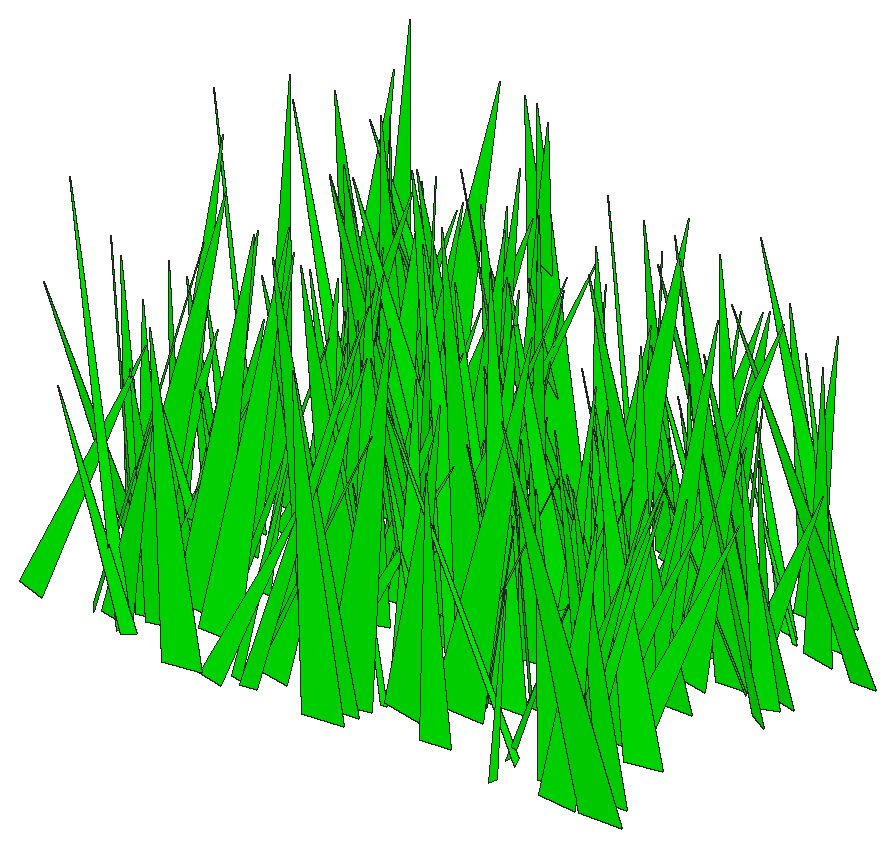
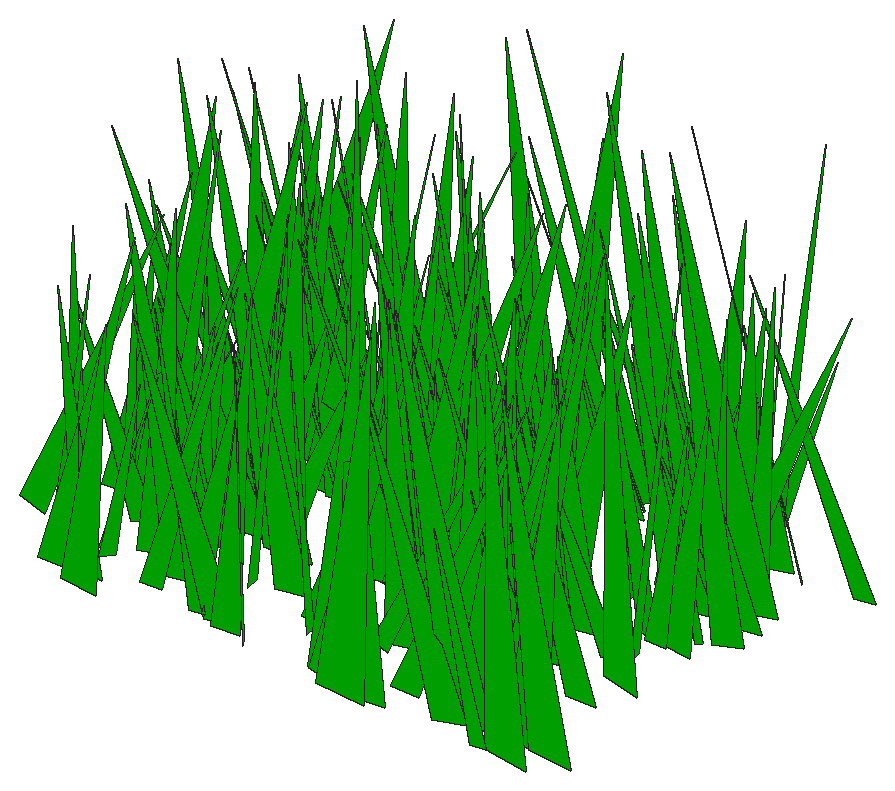
# SketchUp Ruby script. Lengths in inches.
U = 1.inch
M = Sketchup.active_model
def pt(a) = Geom::Point3d.new(a.map { |v| v * U })
def face(e, loops, mat)
  f = e.add_face(loops[0].map { |a| pt(a) })
  loops[1..].each { |l| e.add_face(l.map { |a| pt(a) }).erase! }
  f.material = f.back_material = mat if mat
  f
end
# faces: each face lists its corners as indices into pts; further lists are holes
def faces(e, pts, list, mat = nil) = list.each { |f| face(e, (f[0].is_a?(Array) ? f : [f]).map { |l| l.map { |i| pts[i] } }, mat) }
# xy, xz, yz: faces in a plane at the given z, y or x. An outline is a flat list of corners, or four numbers for a rectangle; further outlines are holes
def ring(l) = l.size == 4 ? [[l[0], l[1]], [l[2], l[1]], [l[2], l[3]], [l[0], l[3]]] : l.each_slice(2).to_a
def flat(e, list, mat, &to3) = list.each { |f| face(e, (f[0].is_a?(Array) ? f : [f]).map { |l| ring(l).map { |u, v| to3.(u, v) } }, mat) }
def xy(e, z, list, mat = nil) = flat(e, list, mat) { |x, y| [x, y, z] }
def xz(e, y, list, mat = nil) = flat(e, list, mat) { |x, z| [x, y, z] }
def yz(e, x, list, mat = nil) = flat(e, list, mat) { |y, z| [x, y, z] }
def lines(e, pts, list) = list.each { |a, b| e.add_line(pt(pts[a]), pt(pts[b])) }
# prism: a flat outline (further loops are holes) pulled along v
def prism(e, loops, v, mat = nil)
  f = face(e, loops, mat); d = Geom::Vector3d.new(v.map { |x| x * U })
  f.pushpull(f.normal.samedirection?(d) ? d.length : -d.length)
end
def box(e, o, s, mat = nil) = prism(e, [[o, [o[0] + s[0], o[1], o[2]], [o[0] + s[0], o[1] + s[1], o[2]], [o[0], o[1] + s[1], o[2]]]], [0, 0, s[2]], mat)
def at(x, y, z, deg = 0) = Geom::Transformation.translation(pt([x, y, z])) * Geom::Transformation.rotation(ORIGIN, Z_AXIS, deg.degrees)
def axes(o, x, y, z) = Geom::Transformation.new([*x, 0, *y, 0, *z, 0, *pt(o).to_a, 1])
def part(name) = M.definitions.add(name)
# library, detail: a bought-in or finely detailed component or shape, given as its bounding box
def library(name, o, s) = part(name).tap { |d| box(d.entities, o, s) }
def detail(e, o, s) = box(e.add_group.entities, o, s)
def put(e, d, t, mat = nil) = e.add_instance(d, t).tap { |i| i.material = mat if mat }
def group(e, t, mat = nil) = e.add_group.tap { |g| g.transformation = t; g.material = mat if mat }.entities
root = M.entities
M.materials.add("[0065_Lime]").color = [0, 255, 0]
c1 = part("fur_instance\#9")
p = [[0.8125,0,1.79],[0.67,-0.02,1.48],[0,-0.11,0],[0,0.11,0]]
faces(c1.entities,p,[[0,1,2,3]])
put(root,c1,axes([71.11,32.47,1.48],[1.31504,-1.01474,1.32526],[7.31505,0.21385,0.68416],[-1.1376,0.20206,5.93131]),"[0065_Lime]")
put(root,c1,axes([70.0625,32.63,1.48],[3.16788,1.04057,0.61952],[-7.4056,0.45235,-0.40482],[-0.75859,-0.07058,6.53906]),"[0065_Lime]")
put(root,c1,axes([71.28,25.28,1.48],[-0.49526,-0.70471,1.4178],[5.29109,-0.04513,0.47119],[-0.43981,0.25059,4.072]),"[0065_Lime]")
put(root,c1,axes([71.29,21.32,1.48],[6.28785,0.11215,2.7973],[-0.35978,1.00228,-0.81143],[-3.51199,0.09812,5.0914]),"[0065_Lime]")
put(root,c1,axes([72.81,20.59,1.48],[-4.84312,-0.62522,0.45458],[4.4821,-0.6712,0.6608],[-0.1432,0.13709,5.30862]),"[0065_Lime]")
put(root,c1,axes([71.03,21.84,1.48],[5.05659,-0.53702,2.1019],[3.79865,0.79038,0.72027],[-2.61785,0.10959,5.10514]),"[0065_Lime]")
put(root,c1,axes([68.77,19.51,1.48],[4.73607,0.58974,0.54638],[-4.24651,0.65059,0.82395],[0.17935,-0.16892,5.08094]),"[0065_Lime]")
put(root,c1,axes([71.95,26.32,1.48],[-8.48103,0.12944,2.12396],[-0.61842,-1.24092,0.90029],[2.69894,0.12241,6.8805]),"[0065_Lime]")
put(root,c1,axes([71.07,33.45,1.48],[4.07033,1.04268,1.70118],[-7.52786,0.60923,-0.5954],[-1.66314,-0.20574,6.8584]),"[0065_Lime]")
put(root,c1,axes([70.23,24.1,1.48],[7.45772,-0.59253,2.41896],[4.64223,1.0911,-0.5137],[-2.25262,0.28689,6.94979]),"[0065_Lime]")
put(root,c1,axes([71.17,27.95,1.48],[5.96669,0.87695,2.17628],[-6.27778,0.90317,-0.80728],[-2.58765,-0.16905,6.97663]),"[0065_Lime]")
put(root,c1,axes([72.04,32.25,1.48],[0.25386,-0.75206,1.27851],[5.50134,0.0703,0.66302],[-0.9221,0.21239,4.3076]),"[0065_Lime]")
put(root,c1,axes([72.67,19.22,1.48],[-4.15449,0.31536,0.77462],[-2.40098,-0.57513,-0.67404],[0.42308,-0.16713,3.78127]),"[0065_Lime]")
put(root,c1,axes([71.95,25.34,1.48],[3.10497,-0.43272,1.84859],[3.21889,0.51771,0.48359],[-2.07044,0.15594,3.52411]),"[0065_Lime]")
put(root,c1,axes([71.68,22.82,1.48],[4.8907,0.49632,1.94087],[-3.40285,0.76194,-0.85566],[-2.56705,-0.06443,4.83198]),"[0065_Lime]")
put(root,c1,axes([72.34,19.4,1.48],[-8.64109,0.1221,2.44965],[-1.21349,-1.27456,-0.70341],[2.88998,-0.1701,7.02912]),"[0065_Lime]")
put(root,c1,axes([70.38,23.06,1.48],[0.93197,0.76973,0.26058],[-5.4343,0.12315,0.66989],[0.76009,-0.06333,4.46986]),"[0065_Lime]")
put(root,c1,axes([70.94,31.95,1.48],[0.54433,0.53862,1.59453],[-4.28288,0.03946,0.52074],[0.43863,-0.28314,3.10583]),"[0065_Lime]")
put(root,c1,axes([70.98,24.51,1.48],[3.81899,0.20071,1.17784],[-1.81606,0.5314,0.86171],[-0.91588,-0.21679,3.20267]),"[0065_Lime]")
put(root,c1,axes([70.98,31.86,1.48],[-0.66186,-0.82891,0.88827],[5.88182,-0.12005,-0.85414],[1.18088,0.13336,4.75225]),"[0065_Lime]")
put(root,c1,axes([72.12,32.28,1.48],[-2.30581,0.56203,0.7001],[-3.98197,-0.34017,0.47345],[0.93939,-0.06239,3.72537]),"[0065_Lime]")
put(root,c1,axes([72.6875,20.4,1.48],[1.18339,0.93993,0.30109],[-6.60693,0.17248,-0.8617],[-1.1084,-0.02462,5.45783]),"[0065_Lime]")
put(root,c1,axes([70.65,23.57,1.48],[3.30012,0.38045,0.41179],[-2.74444,0.44474,0.78362],[0.23403,-0.14935,3.38258]),"[0065_Lime]")
put(root,c1,axes([72.34,32.04,1.48],[6.11772,0.32407,2.61673],[-2.78615,0.94364,0.39383],[-2.81158,-0.22997,5.30348]),"[0065_Lime]")
put(root,c1,axes([70.75,22.13,1.48],[5.9783,-0.91796,1.63314],[6.78643,0.84165,-0.58455],[-0.80738,0.27735,7.17927]),"[0065_Lime]")
put(root,c1,axes([73.11,20.22,1.48],[1.39656,-0.78388,0.40984],[5.50287,0.20563,0.77201],[-1.0449,0.03523,4.6135]),"[0065_Lime]")
put(root,c1,axes([71.66,24.4375,1.48],[2.25771,-0.74217,0.60841],[5.33057,0.30957,-0.43405],[0.20209,0.12595,4.65205]),"[0065_Lime]")
put(root,c1,axes([71.875,19.65,1.48],[-0.08074,-0.72173,0.01146],[5.03229,-0.01151,-0.83628],[1.02821,-0.00033,4.09385]),"[0065_Lime]")
put(root,c1,axes([74.12,21.72,1.48],[-3.14063,0.42918,0.55548],[-3.12964,-0.43128,-0.54179],[0.0139,-0.13403,3.52203]),"[0065_Lime]")
put(root,c1,axes([72.69,28.5,1.48],[3.70073,-0.17932,1.47637],[1.71458,0.54593,-0.62163],[-1.40824,0.19345,3.12291]),"[0065_Lime]")
put(root,c1,axes([72.17,33.36,1.48],[2.89286,0.41494,0.9781],[-3.1635,0.40198,0.47634],[-0.39735,-0.17946,3.32858]),"[0065_Lime]")
put(root,c1,axes([70.89,19.82,1.48],[8.6912,0.11024,1.35526],[-0.9364,1.23708,0.60131],[-1.58577,-0.1263,7.07277]),"[0065_Lime]")
put(root,c1,axes([73.49,31.82,1.48],[-0.1084,-0.97511,0.82499],[6.99594,-0.00506,0.40785],[-0.49087,0.14324,5.63054]),"[0065_Lime]")
put(root,c1,axes([73.34,29.99,1.48],[0.5857,-1.06717,0.33922],[7.58064,0.0867,0.47952],[-0.62062,0.05187,6.17727]),"[0065_Lime]")
put(root,c1,axes([72.37,25.13,1.48],[-4.30663,-0.44805,3.2719],[4.32555,-0.71402,0.49066],[2.76344,0.41938,4.33101]),"[0065_Lime]")
put(root,c1,axes([71.98,21.87,1.48],[2.87091,-0.51429,0.29602],[3.67469,0.39832,-0.39096],[0.15592,0.08183,3.76342]),"[0065_Lime]")
put(root,c1,axes([72.13,23.14,1.48],[-3.68002,0.78053,3.50005],[-6.35559,-0.66081,0.51668],[2.99602,-0.44308,5.39518]),"[0065_Lime]")
put(root,c1,axes([73.91,22.57,1.48],[-3.6477,0.2439,1.28318],[-2.11002,-0.52022,-0.65529],[1.02426,-0.20307,3.21986]),"[0065_Lime]")
put(root,c1,axes([74.97,29.85,1.48],[3.10762,0.62386,3.33133],[-5.14734,0.61217,-0.66452],[-3.16059,-0.38357,4.35774]),"[0065_Lime]")
put(root,c1,axes([72.67,30.68,1.48],[3.63008,0.43879,0.15845],[-3.02235,0.50263,-0.82825],[-0.80887,0.09112,3.80584]),"[0065_Lime]")
put(root,c1,axes([75.91,32.1,1.48],[-6.02316,0.56472,0.70733],[-4.10903,-0.83467,-0.82077],[0.15222,-0.18595,5.83232]),"[0065_Lime]")
put(root,c1,axes([71.52,29.36,1.48],[6.73425,-0.62445,0.14362],[4.39122,0.94071,0.82514],[-0.70506,-0.10545,6.51085]),"[0065_Lime]")
put(root,c1,axes([75.26,27.2,1.48],[-8.18372,0.48597,1.34778],[-3.32068,-1.17248,0.82548],[1.91812,0.04358,7.17944]),"[0065_Lime]")
put(root,c1,axes([73.79,27.36,1.48],[-2.93435,0.51989,1.19615],[-3.67999,-0.45214,0.61195],[1.51947,-0.09103,3.79203]),"[0065_Lime]")
put(root,c1,axes([74.44,29.65,1.48],[2.85353,0.9943,2.37939],[-7.44982,0.46184,-0.55573],[-1.76823,-0.34123,6.18117]),"[0065_Lime]")
put(root,c1,axes([72.51,26.72,1.48],[3.64946,-0.40735,0.4785],[2.95439,0.49542,-0.77576],[0.14704,0.15609,3.71089]),"[0065_Lime]")
put(root,c1,axes([72.32,30.33,1.48],[5.23306,0.58126,0.95209],[-4.2862,0.72543,0.74677],[-0.3315,-0.20377,5.37428]),"[0065_Lime]")
put(root,c1,axes([73.17,32.54,1.48],[1.59918,1.18186,1.17789],[-8.51711,0.20779,0.66467],[0.5449,-0.22074,6.93221]),"[0065_Lime]")
put(root,c1,axes([74.08,26.0625,1.48],[-0.73508,0.85642,0.48475],[-6.09321,-0.11071,0.44068],[0.61148,-0.07366,4.97399]),"[0065_Lime]")
put(root,c1,axes([73.55,28.08,1.48],[-3.02491,-0.55036,1.90452],[3.95137,-0.51335,-0.81853],[2.28233,0.15933,3.94129]),"[0065_Lime]")
put(root,c1,axes([75.13,18.62,1.48],[0.04121,0.92089,1.56543],[-6.78137,0.03783,-0.62755],[-0.81608,-0.26783,5.29379]),"[0065_Lime]")
put(root,c1,axes([73.44,21.57,1.48],[3.24663,-1.05491,2.00022],[7.8962,0.44459,-0.62295],[-0.23778,0.36036,6.62388]),"[0065_Lime]")
put(root,c1,axes([74.45,30.97,1.48],[-2.39424,-0.95797,0.7221],[6.75796,-0.3522,-0.83152],[1.26296,0.06856,5.81829]),"[0065_Lime]")
put(root,c1,axes([73.11,24,1.48],[5.73473,-0.05303,0.79258],[0.52989,0.8059,-0.72983],[-0.9006,0.13648,4.61748]),"[0065_Lime]")
put(root,c1,axes([74.28,29.27,1.48],[-0.46338,1.01702,0.52612],[-7.23713,-0.07278,0.4968],[0.65311,-0.08487,5.87834]),"[0065_Lime]")
put(root,c1,axes([74.23,23.58,1.48],[3.72406,-0.17672,1.16654],[1.54448,0.53878,-0.52732],[-1.11935,0.15547,3.15348]),"[0065_Lime]")
put(root,c1,axes([74.375,27.13,1.48],[3.50733,0.79291,0.69174],[-5.61549,0.50452,-0.5399],[-1.015,-0.05135,5.37724]),"[0065_Lime]")
put(root,c1,axes([75.98,24.51,1.48],[-0.90176,-0.96121,0.4871],[6.8259,-0.11625,0.67401],[-0.74691,0.0981,5.57166]),"[0065_Lime]")
put(root,c1,axes([75.23,29.93,1.48],[2.30693,-0.5219,1.16693],[3.75477,0.36267,0.52389],[-1.3245,0.11912,3.51763]),"[0065_Lime]")
put(root,c1,axes([74.76,24.91,1.48],[4.15362,0.458,0.72632],[-3.13805,0.59649,-0.73038],[-1.25443,0.02434,4.23208]),"[0065_Lime]")
put(root,c1,axes([73.72,32.75,1.48],[3.218,-0.77653,0.66071],[5.56314,0.43377,-0.84399],[0.50052,0.17129,5.13277]),"[0065_Lime]")
put(root,c1,axes([78.17,30.43,1.48],[-5.83788,-0.46117,0.22125],[3.29279,-0.81616,0.48009],[-0.05329,0.09101,5.42637]),"[0065_Lime]")
put(root,c1,axes([76.52,24.84,1.48],[4.31305,-0.62067,2.26086],[4.44197,0.70257,0.85634],[-2.73945,0.162,4.94809]),"[0065_Lime]")
put(root,c1,axes([76.0625,29.91,1.48],[3.01042,-0.54942,1.28467],[3.90462,0.46616,0.62652],[-1.59249,0.10436,3.96467]),"[0065_Lime]")
put(root,c1,axes([74.8,20.78,1.48],[6.79529,-0.77285,2.35553],[5.99639,0.97384,-0.73871],[-1.63688,0.35912,7.07254]),"[0065_Lime]")
put(root,c1,axes([75.37,25.12,1.48],[4.0932,0.26235,1.23612],[-2.19458,0.57978,0.68484],[-0.98942,-0.20067,3.59481]),"[0065_Lime]")
put(root,c1,axes([75.55,24.88,1.48],[5.32177,0.64563,1.08737],[-4.57087,0.76901,-0.49902],[-1.41609,-0.05587,5.69714]),"[0065_Lime]")
put(root,c1,axes([77.3,33.4,1.48],[0.22789,1.11679,1.46084],[-8.09237,0.06049,-0.71444],[-0.95124,-0.24709,6.42783]),"[0065_Lime]")
put(root,c1,axes([76.4,25.09,1.48],[-1.928,-0.83561,0.78754],[5.90862,-0.29017,-0.74615],[1.17836,0.08779,5.02994]),"[0065_Lime]")
put(root,c1,axes([78.49,25.86,1.48],[-2.47415,-1.1779,1.13536],[8.47294,-0.32627,0.87409],[-0.65157,0.22997,7.05533]),"[0065_Lime]")
put(root,c1,axes([77.8,23.2,1.48],[-1.38711,-1.00644,1.66313],[7.4428,-0.17587,0.54093],[-0.2909,0.29934,5.9095]),"[0065_Lime]")
put(root,c1,axes([76.59,33.28,1.48],[-1.07702,-1.0919,1.70475],[7.99318,-0.17982,-0.51815],[0.93989,0.27803,6.36004]),"[0065_Lime]")
put(root,c1,axes([78.02,28.24,1.48],[2.46566,-0.78758,2.73535],[6.19279,0.44305,0.58117],[-2.09099,0.38345,4.94669]),"[0065_Lime]")
put(root,c1,axes([76.4375,29.61,1.48],[3.1994,-0.55741,0.00222],[3.9451,0.44716,0.43172],[-0.41482,-0.04652,4.12284]),"[0065_Lime]")
put(root,c1,axes([78.48,28.57,1.48],[-2.10114,-1.10844,1.32766],[8.05154,-0.28169,0.55036],[-0.24809,0.24582,6.61729]),"[0065_Lime]")
put(root,c1,axes([78.14,32.69,1.48],[-1.1822,1.15866,1.08632],[-8.34829,-0.15743,-0.38443],[-0.28458,-0.19501,6.76482]),"[0065_Lime]")
put(root,c1,axes([78.54,25.65,1.48],[-3.16549,-0.70017,1.42934],[5.27691,-0.43337,0.61868],[0.26458,0.26648,4.76175]),"[0065_Lime]")
put(root,c1,axes([76.09,27.26,1.48],[4.57029,0.61363,0.15937],[-4.34545,0.64209,-0.3923],[-0.47459,0.03006,5.12674]),"[0065_Lime]")
put(root,c1,axes([78.46,32.86,1.48],[1.20082,0.55625,1.73094],[-4.22584,0.24512,-0.69982],[-1.53006,-0.24042,3.29128]),"[0065_Lime]")
put(root,c1,axes([77.55,30.02,1.48],[-2.51079,0.95271,0.74865],[-6.73508,-0.36841,0.765],[1.20598,-0.07399,5.831]),"[0065_Lime]")
put(root,c1,axes([76.79,19.1,1.48],[5.48271,-0.0756,1.22071],[0.83045,0.78013,-0.84889],[-1.36088,0.17148,4.39999]),"[0065_Lime]")
put(root,c1,axes([77.82,28.08,1.48],[-4.10817,0.40382,1.36068],[-2.76052,-0.62247,0.67585],[1.85384,-0.03202,4.02172]),"[0065_Lime]")
put(root,c1,axes([76.23,18.59,1.48],[3.20672,0.54972,0.08846],[-3.88914,0.44541,0.53126],[0.43686,-0.06991,4.08014]),"[0065_Lime]")
put(root,c1,axes([77.85,24.07,1.48],[4.72637,-0.81215,1.78479],[5.83099,0.71458,0.67923],[-2.05406,0.15976,6.03497]),"[0065_Lime]")
put(root,c1,axes([77.27,29.98,1.48],[5.19341,0.77607,2.53629],[-6.15624,0.753,0.61976],[-1.52502,-0.39688,6.13539]),"[0065_Lime]")
put(root,c1,axes([79.35,26.52,1.48],[-1.44303,1.24728,0.4097],[-8.85468,-0.19519,-0.72326],[-0.7986,-0.0896,7.27908]),"[0065_Lime]")
put(root,c1,axes([80.625,25.64,1.48],[-6.36802,0.83775,0.95074],[-6.07404,-0.8829,-0.84895],[0.12744,-0.21946,7.04467]),"[0065_Lime]")
put(root,c1,axes([77.67,25.53,1.48],[2.43463,0.56758,0.166],[-4.00552,0.34302,-0.43141],[-0.55934,0.0141,3.81191]),"[0065_Lime]")
put(root,c1,axes([76.99,25.875,1.48],[6.442,0.82447,1.21552],[-5.84842,0.92667,-0.55422],[-1.5669,-0.06915,7.066]),"[0065_Lime]")
put(root,c1,axes([79.85,27.45,1.48],[-2.8246,0.72539,0.65705],[-5.21575,-0.38372,-0.63997],[-0.31243,-0.15225,4.74356]),"[0065_Lime]")
put(root,c1,axes([77.38,29.06,1.48],[1.20081,-0.95529,0.35094],[6.78391,0.16211,-0.5713],[0.61833,0.07659,5.58633]),"[0065_Lime]")
put(root,c1,axes([80.34,30.59,1.48],[-2.94035,-0.85872,0.21678],[6.10183,-0.40884,0.49118],[-0.42947,0.07043,5.49441]),"[0065_Lime]")
put(root,c1,axes([77.02,24.84,1.48],[6.00998,-0.26469,0.74113],[1.97426,0.84631,-0.46447],[-0.69329,0.1155,5.10198]),"[0065_Lime]")
put(root,c1,axes([79.59,24.31,1.48],[-3.01184,-0.78611,0.04261],[5.56333,-0.42171,-0.52305],[0.59092,-0.03639,5.14157]),"[0065_Lime]")
put(root,c1,axes([77.45,19.8125,1.48],[4.24134,0.87462,0.88458],[-6.31828,0.58879,0.53672],[-0.0591,-0.17855,6.10304]),"[0065_Lime]")
put(root,c1,axes([78.88,24.94,1.48],[8.18641,0.45923,2.77913],[-3.24905,1.2438,-0.55473],[-3.43479,-0.08202,7.14846]),"[0065_Lime]")
put(root,c1,axes([80.14,19.4,1.48],[-1.56496,-1.27543,1.64642],[9.29462,-0.20509,0.52163],[-0.30396,0.29528,7.47381]),"[0065_Lime]")
put(root,c1,axes([78.42,27.79,1.48],[2.1372,-1.05035,1.52844],[7.70739,0.29086,-0.43277],[0.01093,0.27441,6.30894]),"[0065_Lime]")
put(root,c1,axes([77.2,28.8125,1.48],[6.7204,0.28868,0.80784],[-2.17705,0.94119,0.71274],[-0.68365,-0.1594,5.67157]),"[0065_Lime]")
put(root,c1,axes([77.16,19.35,1.48],[6.50746,0.12255,0.4227],[-0.94033,0.90615,0.77512],[-0.38263,-0.14273,5.28403]),"[0065_Lime]")
put(root,c1,axes([77.4,18.9,1.48],[8.88346,-0.25502,1.40947],[1.9739,1.26326,-0.57253],[-1.54916,0.14725,7.35292]),"[0065_Lime]")
put(root,c1,axes([77.09,29.02,1.48],[6.94547,0.46074,0.59183],[-3.35087,0.96654,0.80493],[-0.22813,-0.16959,6.19537]),"[0065_Lime]")
put(root,c1,axes([80.48,27.43,1.48],[-0.50193,1.08997,2.00513],[-8.11919,-0.04279,-0.56527],[-0.56898,-0.35089,6.29738]),"[0065_Lime]")
put(root,c1,axes([80.31,18.73,1.48],[0.78038,-0.93487,2.09352],[7.07381,0.14838,0.4756],[-0.9208,0.34757,5.42795]),"[0065_Lime]")
put(root,c1,axes([77.96,22.8,1.48],[4.2754,0.34372,0.0692],[-2.43719,0.59563,0.48947],[0.22559,-0.0793,3.97663]),"[0065_Lime]")
put(root,c1,axes([80.5,25.34,1.48],[-3.64389,-0.64071,0.36373],[4.44945,-0.51404,-0.84863],[1.09207,-0.0435,4.67127]),"[0065_Lime]")
put(root,c1,axes([79.66,24.97,1.48],[2.71711,0.51161,0.08174],[-3.60734,0.38043,-0.45028],[-0.50341,0.0353,3.66781]),"[0065_Lime]")
put(root,c1,axes([82.38,26.49,1.48],[-3.80518,0.31175,0.06817],[-2.17515,-0.51879,-0.83211],[-0.44494,-0.12997,3.4849]),"[0065_Lime]")
put(root,c1,axes([81.17,20.51,1.48],[-4.23229,0.07919,0.94334],[-0.43802,-0.61422,0.42751],[1.21272,0.05451,3.44657]),"[0065_Lime]")
put(root,c1,axes([80.3,31.02,1.48],[-5.19573,0.13295,2.0938],[-0.59019,-0.81092,0.75638],[2.6782,0.07922,4.22866]),"[0065_Lime]")
put(root,c1,axes([81.71,23.66,1.48],[-6.03137,0.86442,0.93728],[-6.06601,-0.86275,0.83536],[1.5408,-0.01286,6.95768]),"[0065_Lime]")
put(root,c1,axes([81.83,24.86,1.48],[-5.52923,0.71146,0.89133],[-4.98086,-0.79203,0.74095],[1.42388,-0.00781,6.05314]),"[0065_Lime]")
put(root,c1,axes([82.7,26.24,1.48],[-8.79981,-0.33642,1.9718],[2.6105,-1.272,0.4361],[2.1894,0.16449,7.40524]),"[0065_Lime]")
put(root,c1,axes([78.95,24.96,1.48],[5.87801,-0.65777,0.69465],[4.75829,0.81224,-0.86787],[0.00767,0.19203,6.05022]),"[0065_Lime]")
put(root,c1,axes([81.51,21.25,1.48],[-2.68263,0.88201,0.59883],[-6.22686,-0.38809,0.6978],[1.08044,-0.04672,5.50842]),"[0065_Lime]")
put(root,c1,axes([82.53,21.22,1.48],[-4.2119,0.42275,0.13084],[-2.94497,-0.58589,0.70894],[0.63586,0.08675,4.15014]),"[0065_Lime]")
put(root,c1,axes([80.4,19.81,1.48],[4.99595,-1.0753,0.65218],[7.62429,0.70992,0.57921],[-1.03552,0.03914,7.41107]),"[0065_Lime]")
put(root,c1,axes([81.42,32.75,1.48],[5.73346,0.0821,1.97299],[-0.41561,0.87369,-0.41917],[-2.46008,0.04374,4.66904]),"[0065_Lime]")
put(root,c1,axes([82.28,23.53,1.48],[-4.67638,-0.97872,2.928],[7.72615,-0.67539,0.59951],[1.3329,0.48114,6.79762]),"[0065_Lime]")
put(root,c1,axes([81.05,26.625,1.48],[4.00896,-0.24107,1.25733],[2.01063,0.57842,-0.52539],[-1.13579,0.17304,3.50787]),"[0065_Lime]")
put(root,c1,axes([79.93,24.49,1.48],[3.25076,0.37691,0.23694],[-2.65603,0.43579,0.88147],[0.47421,-0.14291,3.31286]),"[0065_Lime]")
put(root,c1,axes([82.25,32.56,1.48],[-4.50206,-0.77205,1.30374],[5.46943,-0.66477,-0.69479],[1.68579,0.09496,5.73595]),"[0065_Lime]")
put(root,c1,axes([82.9,25.34,1.48],[-4.81216,0.39498,1.45809],[-3.11805,-0.68977,-0.54751],[1.17988,-0.21191,4.49994]),"[0065_Lime]")
put(root,c1,axes([81.82,24.17,1.48],[6.08596,-0.63255,2.48212],[5.06476,0.89364,-0.58526],[-1.98087,0.34147,6.12955]),"[0065_Lime]")
put(root,c1,axes([83.39,29.875,1.48],[-7.8263,0.11845,2.10005],[-0.52084,-1.1515,0.89204],[2.66549,0.12278,6.34039]),"[0065_Lime]")
put(root,c1,axes([81.9,20.5,1.48],[-1.78123,-0.8748,1.98609],[6.47492,-0.31437,-0.79777],[1.67164,0.28554,5.20636]),"[0065_Lime]")
put(root,c1,axes([82.93,25.25,1.48],[1.64022,-0.61747,0.90012],[4.44871,0.25088,0.40338],[-0.86217,0.11983,3.79387]),"[0065_Lime]")
put(root,c1,axes([84.38,27.1875,1.48],[-1.99881,-0.61645,0.45092],[4.36064,-0.26061,0.8505],[-0.73338,0.13052,3.82803]),"[0065_Lime]")
put(root,c1,axes([82.14,29.57,1.48],[-0.38334,0.81119,1.51945],[-5.97418,-0.09644,0.72797],[1.06066,-0.25,4.64945]),"[0065_Lime]")
put(root,c1,axes([82.78,25.68,1.48],[-6.96081,-0.76138,2.73516],[5.43068,-1.07441,-0.87745],[3.34264,0.16005,7.12133]),"[0065_Lime]")
put(root,c1,axes([82.02,24.67,1.48],[8.19393,0.07153,1.85396],[-0.73417,1.18811,0.61086],[-2.21698,-0.12908,6.6499]),"[0065_Lime]")
put(root,c1,axes([83.79,19.64,1.48],[0.9533,0.7566,0.98881],[-5.46341,0.15407,-0.46532],[-0.78782,-0.15292,4.42344]),"[0065_Lime]")
put(root,c1,axes([84.57,22.9,1.48],[-5.13713,-0.0362,0.93061],[0.15415,-0.73692,-0.39765],[1.16256,-0.06227,4.16492]),"[0065_Lime]")
put(root,c1,axes([84.15,27.48,1.48],[-4.01227,0.9967,1.0971],[-7.11683,-0.58249,0.51163],[1.21701,-0.12036,6.6089]),"[0065_Lime]")
put(root,c1,axes([84.04,22.58,1.48],[-5.45865,0.93269,2.04946],[-6.80891,-0.81424,0.41777],[2.01092,-0.22519,6.97782]),"[0065_Lime]")
put(root,c1,axes([84.1,23.69,1.48],[4.14383,-0.00014,1.77729],[-0.39725,0.64725,0.61458],[-2.14856,-0.11995,3.31414]),"[0065_Lime]")
put(root,c1,axes([86.33,20.28,1.48],[-7.25527,-0.02961,0.42537],[0.14613,-1.01481,-0.71814],[0.54454,-0.12221,5.86018]),"[0065_Lime]")
put(root,c1,axes([83.49,22.43,1.48],[3.91452,0.02282,0.95946],[-0.32997,0.56805,0.43797],[-1.14404,-0.08575,3.15662]),"[0065_Lime]")
put(root,c1,axes([85.39,24.28,1.48],[-6.68801,0.59707,1.99811],[-4.63555,-0.96013,-0.65217],[1.61261,-0.28371,6.41212]),"[0065_Lime]")
put(root,c1,axes([82.67,32.27,1.48],[2.21604,0.80266,0.82189],[-5.76107,0.28676,0.89344],[0.67832,-0.1868,4.90303]),"[0065_Lime]")
put(root,c1,axes([85.64,31.79,1.48],[-5.59292,-0.62313,0.46351],[4.36069,-0.78857,-0.70996],[0.98716,-0.04703,5.76229]),"[0065_Lime]")
put(root,c1,axes([85.15,30.14,1.48],[-0.52586,0.61868,1.07743],[-4.54489,-0.04162,-0.66689],[-0.69525,-0.19589,3.54458]),"[0065_Lime]")
put(root,c1,axes([83.61,32.19,1.48],[4.92793,0.40113,1.6358],[-3.23366,0.7087,0.62197],[-1.31792,-0.23896,4.59049]),"[0065_Lime]")
put(root,c1,axes([82.61,21.59,1.48],[5.87521,0.19062,0.22693],[-1.30487,0.81915,-0.70451],[-0.46408,0.10998,4.85384]),"[0065_Lime]")
put(root,c1,axes([83.14,21.53,1.48],[3.88855,-1.10402,1.40949],[8.04558,0.53467,-0.65258],[-0.03246,0.26828,7.10082]),"[0065_Lime]")
put(root,c1,axes([83.62,27.92,1.48],[3.88757,1.1708,1.63211],[-8.56622,0.5403,0.51263],[-0.26184,-0.29323,7.4612]),"[0065_Lime]")
put(root,c1,axes([83.78,27.33,1.48],[3.6764,-0.27732,0.76764],[2.17106,0.49434,-0.8953],[-0.26831,0.20021,3.27386]),"[0065_Lime]")
put(root,c1,axes([86.26,24.98,1.48],[-0.88395,0.62375,0.19608],[-4.37337,-0.11582,-0.69876],[-0.79747,-0.05622,3.61467]),"[0065_Lime]")
put(root,c1,axes([84.55,24.41,1.48],[5.81738,-0.49626,1.27866],[3.47487,0.84618,0.54453],[-1.69377,0.03155,5.50881]),"[0065_Lime]")
put(root,c1,axes([86.4,30.07,1.48],[-4.62986,-0.18598,0.80417],[1.15266,-0.6598,-0.72227],[1.1834,-0.08494,3.84967]),"[0065_Lime]")
put(root,c1,axes([85.05,30.13,1.48],[1.35889,0.54956,0.32425],[-3.91675,0.18418,0.4003],[0.3371,-0.07534,3.34391]),"[0065_Lime]")
put(root,c1,axes([84.24,24.66,1.48],[5.57856,-0.00458,0.5405],[-0.04676,0.78384,0.54211],[-0.66364,-0.09377,4.50526]),"[0065_Lime]")
put(root,c1,axes([86.66,29.52,1.48],[0.46992,-0.70398,0.38878],[4.9535,0.07662,0.68733],[-0.88909,0.05478,4.03489]),"[0065_Lime]")
put(root,c1,axes([87.43,25.11,1.48],[-6.54962,0.03314,1.17067],[-0.05837,-0.93568,0.67152],[1.45724,0.11147,5.28854]),"[0065_Lime]")
put(root,c1,axes([86.29,28.53,1.48],[3.64418,0.53181,1.5893],[-3.85317,0.56561,-0.4963],[-1.81499,-0.13299,4.24468]),"[0065_Lime]")
put(root,c1,axes([86.74,30.2,1.48],[-4.96642,0.82987,1.23208],[-5.88439,-0.72428,0.6533],[1.59601,-0.08799,6.2426]),"[0065_Lime]")
put(root,c1,axes([86.62,28.59,1.48],[1.53018,-0.65137,0.39111],[4.50972,0.22489,0.87668],[-1.17541,0.01487,3.87272]),"[0065_Lime]")
put(root,c1,axes([84.94,23.08,1.48],[2.64141,0.61967,0.48742],[-4.44406,0.36202,0.51199],[0.23804,-0.11745,4.14985]),"[0065_Lime]")
put(root,c1,axes([87.82,25.66,1.48],[-4.60372,-0.992,1.70856],[7.34986,-0.64137,0.62522],[0.47905,0.307,6.82693]),"[0065_Lime]")
put(root,c1,axes([87.05,24.09,1.48],[-5.11667,0.1241,1.20416],[-0.6623,-0.74307,0.70407],[1.59149,0.08975,4.16441]),"[0065_Lime]")
put(root,c1,axes([84.98,30.92,1.48],[1.72103,-1.05551,0.2103],[7.4695,0.23605,-0.74445],[0.83527,0.0639,6.224]),"[0065_Lime]")
put(root,c1,axes([86.15,29.74,1.48],[-0.32394,-0.57335,0.37838],[4.0658,-0.05401,-0.43909],[0.57807,0.05855,3.3003]),"[0065_Lime]")
put(root,c1,axes([87.25,33.18,1.48],[-0.28061,0.84105,0.9171],[-6.05967,-0.02259,-0.53265],[-0.61311,-0.16169,4.84471]),"[0065_Lime]")
put(root,c1,axes([85.3,28.58,1.48],[3.79178,-0.40462,0.64091],[2.97876,0.52466,-0.56112],[-0.19801,0.1445,3.83195]),"[0065_Lime]")
put(root,c1,axes([87.79,28.41,1.48],[-7.40123,-0.50282,2.3296],[4.04203,-1.07643,0.71113],[2.16084,0.2913,6.64905]),"[0065_Lime]")
put(root,c1,axes([86.46,19.01,1.48],[3.94969,-0.15008,1.06187],[0.89606,0.58242,0.55313],[-1.42899,-0.0496,3.28183]),"[0065_Lime]")
put(root,c1,axes([88.74,27.99,1.48],[-6.25451,0.30662,0.42661],[-2.13393,-0.8801,0.49669],[0.69486,0.0571,5.36528]),"[0065_Lime]")
put(root,c1,axes([87.74,31.2,1.48],[-3.66746,0.35836,0.1901],[-2.44053,-0.50644,0.83878],[0.77623,0.10088,3.5354]),"[0065_Lime]")
put(root,c1,axes([86.85,23.18,1.48],[-3.92239,0.71951,1.67684],[-5.16908,-0.60345,0.67653],[1.93631,-0.15343,5.20281]),"[0065_Lime]")
put(root,c1,axes([88.28,30.84,1.48],[-4.21527,0.05358,0.4915],[-0.30105,-0.59396,0.46126],[0.64796,0.07258,3.41171]),"[0065_Lime]")
put(root,c1,axes([86,20.37,1.48],[4.05587,-0.14997,0.2109],[0.98979,0.5595,0.73777],[-0.47607,-0.11444,3.33068]),"[0065_Lime]")
put(root,c1,axes([88.79,32.5,1.48],[-6.36237,0.54349,1.46012],[-4.11031,-0.90227,-0.59637],[1.13464,-0.22095,6.02706]),"[0065_Lime]")
put(root,c1,axes([88.9375,27.73,1.48],[-4.32049,-0.06683,0.12785],[0.44829,-0.60147,-0.51127],[0.22341,-0.08546,3.49841]),"[0065_Lime]")
put(root,c1,axes([87.99,19.95,1.48],[1.67574,0.77503,1.37732],[-5.62629,0.27439,-0.64476],[-1.27802,-0.19175,4.64438]),"[0065_Lime]")
put(root,c1,axes([85.22,27.59,1.48],[3.9163,1.06753,0.05177],[-7.55269,0.54596,0.77946],[0.8228,-0.0696,6.90852]),"[0065_Lime]")
put(root,c1,axes([88.04,22.98,1.48],[2.70658,0.7327,1.57635],[-5.29376,0.43229,-0.7192],[-1.70899,-0.17867,4.7243]),"[0065_Lime]")
put(root,c1,axes([87.54,24.5,1.48],[5.15379,-0.7959,2.01065],[5.7849,0.78043,0.5409],[-2.17412,0.18985,6.2055]),"[0065_Lime]")
put(root,c1,axes([88.74,27.75,1.48],[-1.78468,-1.20142,1.61987],[8.77482,-0.23548,0.54403],[-0.2658,0.29282,7.0837]),"[0065_Lime]")
put(root,c1,axes([86.99,25.7,1.48],[3.69888,-0.52446,0.02833],[3.6741,0.51282,0.72549],[-0.65768,-0.0848,4.21223]),"[0065_Lime]")
put(root,c1,axes([87.58,32.34,1.48],[3.18093,0.72307,0.90959],[-5.16884,0.46381,-0.39509],[-1.00623,-0.09673,4.90491]),"[0065_Lime]")
put(root,c1,axes([88.79,20.875,1.48],[-5.29492,-0.53682,2.06984],[4.33422,-0.76445,0.69244],[1.5114,0.31154,5.26563]),"[0065_Lime]")
put(root,c1,axes([86.71,26.27,1.48],[7.11656,-0.72968,1.04568],[5.08822,1.01609,0.84725],[-1.65166,-0.01375,7.11566]),"[0065_Lime]")
put(root,c1,axes([87.63,28.86,1.48],[5.62619,-0.03658,1.49291],[-0.0702,0.81934,0.84786],[-1.85241,-0.14217,4.50218]),"[0065_Lime]")
put(root,c1,axes([87.27,27.125,1.48],[-2.09372,-0.71807,2.90223],[5.86949,-0.40504,-0.5565],[2.09601,0.41697,4.45744]),"[0065_Lime]")
put(root,c1,axes([89.35,22.41,1.48],[-3.44413,0.84273,1.5615],[-6.27908,-0.48284,-0.43147],[0.47581,-0.27175,5.60893]),"[0065_Lime]")
put(root,c1,axes([86.6,24.2,1.48],[4.4862,-0.41605,0.25784],[2.97754,0.62581,-0.43984],[0.03515,0.08794,4.35005]),"[0065_Lime]")
put(root,c1,axes([90.37,19.13,1.48],[-3.4451,-1.0646,0.56352],[7.60549,-0.47925,0.42484],[-0.19088,0.11893,6.75651]),"[0065_Lime]")
put(root,c1,axes([89.55,31.31,1.48],[-5.48612,0.24577,1.31846],[-1.66674,-0.80382,0.43227],[1.70542,0.00502,4.66379]),"[0065_Lime]")
put(root,c1,axes([88.6875,20.72,1.48],[-1.23783,-0.62481,0.72845],[4.47115,-0.19003,-0.43468],[0.76297,0.0999,3.72912]),"[0065_Lime]")
put(root,c1,axes([90.04,27.91,1.48],[-4.92234,-0.77738,0.46742],[5.48118,-0.69629,-0.61309],[0.94479,-0.0106,5.9921]),"[0065_Lime]")
put(root,c1,axes([86.71,21.56,1.48],[7.00951,0.29567,0.76785],[-2.20453,0.98367,0.6231],[-0.6771,-0.14188,5.92027]),"[0065_Lime]")
put(root,c1,axes([91.37,30.18,1.48],[-5.64635,-0.68209,0.60339],[4.91012,-0.78228,0.76829],[-0.06083,0.16854,6.00781]),"[0065_Lime]")
put(root,c1,axes([90.125,20.05,1.48],[2.97792,0.6592,2.49111],[-5.15977,0.51257,-0.46396],[-2.18249,-0.31236,4.4959]),"[0065_Lime]")
put(root,c1,axes([87.73,24.35,1.48],[2.51238,0.64519,0.26177],[-4.54024,0.33892,0.84019],[0.75641,-0.10869,4.17365]),"[0065_Lime]")
put(root,c1,axes([90.33,26.57,1.48],[-4.97757,-0.36429,0.74647],[2.43714,-0.70785,-0.823],[1.27417,-0.06918,4.49027]),"[0065_Lime]")
put(root,c1,axes([89.5,28.0625,1.48],[-3.80589,-0.4261,1.16658],[2.9074,-0.57104,-0.71329],[1.673,0.02305,3.89343]),"[0065_Lime]")
put(root,c1,axes([89.65,19.59,1.48],[2.69705,-0.41329,0.79988],[2.76517,0.40339,0.81523],[-1.40409,0.00055,3.14194]),"[0065_Lime]")
put(root,c1,axes([88.74,19.14,1.48],[-0.93747,0.76197,2.41157],[-6.04141,-0.20176,0.5823],[1.30204,-0.38756,4.43818]),"[0065_Lime]")
put(root,c1,axes([89.38,30.55,1.48],[-3.225,-0.69116,1.79322],[5.13123,-0.50421,-0.40631],[1.65053,0.21702,4.76696]),"[0065_Lime]")
put(root,c1,axes([88.07,21.06,1.48],[6.07675,-0.24002,1.15251],[1.93431,0.85734,-0.76511],[-1.08793,0.18368,5.07714]),"[0065_Lime]")
put(root,c1,axes([88.2,28.97,1.48],[2.02288,-0.55251,0.69663],[3.97627,0.25373,-0.89643],[0.61874,0.1758,3.48324]),"[0065_Lime]")
put(root,c1,axes([88.13,20.5,1.48],[5.86538,0.39639,1.34876],[-3.11228,0.82348,0.84539],[-1.01029,-0.23551,5.22614]),"[0065_Lime]")
put(root,c1,axes([90.05,27.33,1.48],[2.82915,-0.55623,1.63528],[4.07219,0.45856,0.56514],[-1.76861,0.16605,3.9171]),"[0065_Lime]")
